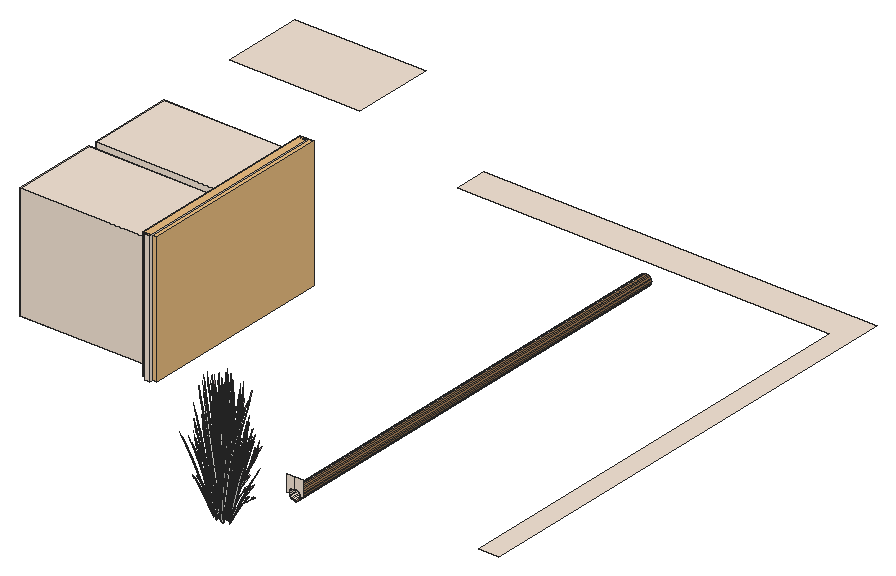
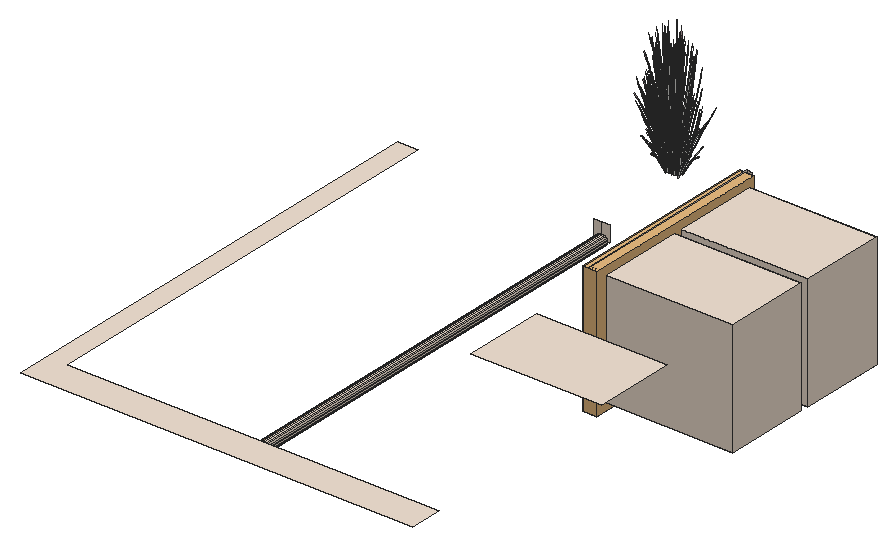
# SketchUp Ruby script. Lengths in inches.
U = 1.inch
M = Sketchup.active_model
def pt(a) = Geom::Point3d.new(a.map { |v| v * U })
def face(e, loops, mat)
  f = e.add_face(loops[0].map { |a| pt(a) })
  loops[1..].each { |l| e.add_face(l.map { |a| pt(a) }).erase! }
  f.material = f.back_material = mat if mat
  f
end
# faces: each face lists its corners as indices into pts; further lists are holes
def faces(e, pts, list, mat = nil) = list.each { |f| face(e, (f[0].is_a?(Array) ? f : [f]).map { |l| l.map { |i| pts[i] } }, mat) }
# xy, xz, yz: faces in a plane at the given z, y or x. An outline is a flat list of corners, or four numbers for a rectangle; further outlines are holes
def ring(l) = l.size == 4 ? [[l[0], l[1]], [l[2], l[1]], [l[2], l[3]], [l[0], l[3]]] : l.each_slice(2).to_a
def flat(e, list, mat, &to3) = list.each { |f| face(e, (f[0].is_a?(Array) ? f : [f]).map { |l| ring(l).map { |u, v| to3.(u, v) } }, mat) }
def xy(e, z, list, mat = nil) = flat(e, list, mat) { |x, y| [x, y, z] }
def xz(e, y, list, mat = nil) = flat(e, list, mat) { |x, z| [x, y, z] }
def yz(e, x, list, mat = nil) = flat(e, list, mat) { |y, z| [x, y, z] }
def lines(e, pts, list) = list.each { |a, b| e.add_line(pt(pts[a]), pt(pts[b])) }
# prism: a flat outline (further loops are holes) pulled along v
def prism(e, loops, v, mat = nil)
  f = face(e, loops, mat); d = Geom::Vector3d.new(v.map { |x| x * U })
  f.pushpull(f.normal.samedirection?(d) ? d.length : -d.length)
end
def box(e, o, s, mat = nil) = prism(e, [[o, [o[0] + s[0], o[1], o[2]], [o[0] + s[0], o[1] + s[1], o[2]], [o[0], o[1] + s[1], o[2]]]], [0, 0, s[2]], mat)
def at(x, y, z, deg = 0) = Geom::Transformation.translation(pt([x, y, z])) * Geom::Transformation.rotation(ORIGIN, Z_AXIS, deg.degrees)
def axes(o, x, y, z) = Geom::Transformation.new([*x, 0, *y, 0, *z, 0, *pt(o).to_a, 1])
def part(name) = M.definitions.add(name)
# library, detail: a bought-in or finely detailed component or shape, given as its bounding box
def library(name, o, s) = part(name).tap { |d| box(d.entities, o, s) }
def detail(e, o, s) = box(e.add_group.entities, o, s)
def put(e, d, t, mat = nil) = e.add_instance(d, t).tap { |i| i.material = mat if mat }
def group(e, t, mat = nil) = e.add_group.tap { |g| g.transformation = t; g.material = mat if mat }.entities
root = M.entities
M.materials.add("C01_Vanilla_Cream").color = [244, 228, 212]
M.materials.add("LightPink_Translucent").color = [144, 107, 117]
M.materials["LightPink_Translucent"].alpha = 0.75
M.materials.add("Wood_Floor_01_1K").color = [146, 111, 76]
c1 = part("blade")
p = [[2.15,0.21,22],[0,0.17,0],[0.09,0.45,0],[2.18,0.31,22],[2.29,0.31,22],[0.38,0.45,0],
  [2.48,0.24,33],[2.49,0.24,33],[2.48,0.22,33]]
faces(c1.entities,p,[[0,1,2,3],[4,5,2,3],[6,3,4,7],[8,0,3,6]])
c2 = part("seeds")
p = [[0.3,-0.1,1.38],[-0.01,-0.03,1.59],[-0.01,-0.03,0.03],[0.14,-0.07,-0.07],[0.29,-0.03,3],[0.15,0.01,3.11]]
faces(c2.entities,p,[[0,1,2,3],[1,0,4,5]],"LightPink_Translucent")
c3 = part("blade with seeds")
put(c3.entities,c1,at(0,0,0))
put(c3.entities,c2,axes([2.4,0.25,30.99],[1.5799,-0.05474,1.17369],[-0.12525,1.92788,0.29478],[-0.07173,-0.02425,1.56792]))
c4 = library("Double casement window",[0,0,0],[5.02,56.42,60])
xy(root,48,[[424.7,306.76,432,306.76,432,480,288,480,288,468,424.7,468],[288,324,290,396]],"C01_Vanilla_Cream")
xy(root,51,[[240,327,290,358.5],[240,361.5,290,393]],"C01_Vanilla_Cream")
xy(root,93,[[240,327,290,358.5],[240,361.5,290,393],[240,423,288,453]],"C01_Vanilla_Cream")
xz(root,306.76,[[354,42,354,48,357,48,357,44,356.48,43.93,356,43.73,355.59,43.41,355.27,43,355.07,42.52,355,42],[359,42,358.93,42.52,358.73,43,358.41,43.41,358,43.73,357.52,43.93,357,44,357,48,360,48,360,42]],"C01_Vanilla_Cream")
xz(root,324,[[288,48,290,96]],"C01_Vanilla_Cream")
xz(root,327,[[240,51,290,93]],"C01_Vanilla_Cream")
xz(root,358.5,[[240,51,290,93]],"C01_Vanilla_Cream")
xz(root,361.5,[[240,51,290,93]],"C01_Vanilla_Cream")
xz(root,393,[[240,51,290,93]],"C01_Vanilla_Cream")
xz(root,396,[[288,48,290,96]],"C01_Vanilla_Cream")
yz(root,240,[[327,51,358.5,93],[361.5,51,393,93]],"C01_Vanilla_Cream")
yz(root,290,[[[324,48,396,96],[327,51,358.5,93],[361.5,51,393,93]]],"C01_Vanilla_Cream")
p = [[357,306.76,40],[356.48,306.76,40.07],[356.48,468,40.07],[357,468,40],[357.52,306.76,40.07],[357.52,468,40.07],
  [356,306.76,40.27],[356,468,40.27],[358,306.76,40.27],[358,468,40.27],[355.59,306.76,40.59],[355.59,468,40.59],
  [358.41,306.76,40.59],[358.41,468,40.59],[355.27,306.76,41],[355.27,468,41],[358.73,306.76,41],[358.73,468,41],
  [355.07,306.76,41.48],[355.07,468,41.48],[358.93,306.76,41.48],[358.93,468,41.48],[355,306.76,42],[355,468,42],
  [359,306.76,42],[359,468,42],[355.07,306.76,42.52],[355.07,468,42.52],[358.93,306.76,42.52],[358.93,468,42.52],
  [355.27,306.76,43],[355.27,468,43],[358.73,306.76,43],[358.73,468,43],[355.59,306.76,43.41],[355.59,468,43.41],
  [358.41,306.76,43.41],[358.41,468,43.41],[356,306.76,43.73],[356,468,43.73],[358,306.76,43.73],[358,468,43.73],
  [356.48,306.76,43.93],[356.48,468,43.93],[357.52,306.76,43.93],[357.52,468,43.93],[357,306.76,44],[357,468,44]]
faces(root,p,[[0,1,2,3],[1,6,7,2],[6,10,11,7],[10,14,15,11],[14,18,19,15],[18,22,23,19],[22,26,27,23],[26,30,31,27],
  [30,34,35,31],[34,38,39,35],[38,42,43,39],[42,46,47,43]],"C01_Vanilla_Cream")
faces(root,p,[[4,0,3,5],[8,4,5,9],[12,8,9,13],[16,12,13,17],[20,16,17,21],[24,20,21,25],[28,24,25,29],[32,28,29,33],
  [36,32,33,37],[40,36,37,41],[44,40,41,45],[46,44,45,47]],"Wood_Floor_01_1K")
put(root,c3,axes([359.9,272.88,51.78],[-0.28012,-0.44611,-0.0912],[0.49717,-0.21923,-0.50621],[0.20951,-0.05886,0.76918]))
put(root,c3,axes([359.88,272.5,51.51],[0.15083,-0.44814,-0.38324],[0.51712,0.15361,-0.29685],[0.2082,-0.04109,0.7333]))
put(root,c3,axes([359.0625,270.67,49.78],[0.34808,-0.49367,0],[0.58235,0.27531,-0.38706],[0.13264,0.0627,1.22783]))
put(root,c3,axes([354.96,271.65,50.91],[0.23093,-0.01116,1.28532],[-0.15319,0.4836,0.10393],[-0.32909,-0.02991,0.54946]))
put(root,c3,axes([356.98,272.78,49.66],[-0.33445,-0.41351,-0.33554],[0.50659,-0.29119,0.16149],[-0.10823,-0.05117,1.07733]))
put(root,c3,axes([357.05,272.2,49.77],[0.24206,0.5509,0.34316],[-0.69162,0.19157,0.13466],[0.00845,-0.10123,1.19142]))
put(root,c3,axes([360.43,272.625,49.49],[-0.35858,0.05912,1.06187],[-0.05708,-0.47061,0.06078],[0.25115,-0.07123,0.60425]))
put(root,c3,axes([361.08,272.21,49.7],[-0.34516,-0.31503,-0.04866],[0.37803,-0.28865,-0.22062],[0.10711,-0.02032,0.72768]))
put(root,c3,axes([356.92,272.63,50.04],[-0.27012,0.44393,0.33554],[-0.56127,-0.21365,-0.16149],[0,-0.10233,1.07733]))
put(root,c3,axes([357.92,272.25,49.65],[0,-0.57005,0],[0.69617,0,0],[0,0,1.34592]))
put(root,c3,axes([358.76,270.93,49.86],[-0.52105,-0.24633,0.37238],[0.31144,-0.44171,0],[0.11867,0.0561,1.18128]))
put(root,c3,axes([359.78,272.66,51.74],[0.48922,-0.21758,-0.53284],[0.27264,0.44789,0.0643],[0.23638,-0.05088,0.75375]))
put(root,c3,axes([356.68,272.94,49.54],[-0.57914,-0.08077,-0.46765],[0.12221,-0.49823,-0.12274],[-0.17283,-0.06037,1.03225]))
put(root,c3,axes([357.59,271.89,49.77],[-0.46162,0.4471,0.34316],[-0.54842,-0.39467,0.13466],[0.11129,-0.04462,1.19142]))
put(root,c3,axes([358.09,272.6875,49.72],[-0.51786,-0.42404,-0.04598],[0.51817,-0.4243,0],[-0.01808,-0.01481,1.31678]))
put(root,c3,axes([356.79,271.15,49.86],[-0.16083,0.48962,0.13232],[-0.58854,-0.13856,0.26315],[0.10167,-0.00238,1.20305]))
put(root,c3,axes([359.71,272.75,51.79],[-0.46269,-0.13744,0.2656],[0.13495,-0.40096,-0.3429],[0.18628,-0.03677,0.65611]))
put(root,c3,axes([354.86,272.01,51.55],[0.15729,-0.44921,0.36002],[0.51712,0.15361,0.29685],[-0.20336,0.027,0.74497]))
put(root,c3,axes([356.54,271.55,49.2],[-0.548,0.19724,0.96696],[-0.17442,-0.56594,0.37572],[0.3365,0.00941,1.09981]))
put(root,c3,axes([358.01,271.7,49.96],[0.1074,-0.43968,0.1086],[0.52474,0.07632,-0.3101],[0.0955,0.04515,0.95058]))
put(root,c3,axes([354.83,271.89,51.55],[-0.20448,-0.33592,0.04823],[0.37288,-0.16442,0.37966],[-0.16437,0.03244,0.57892]))
put(root,c3,axes([357.11,272.74,49.77],[0.70367,0.1038,0.34316],[-0.1432,0.58624,0.13466],[-0.10283,-0.05661,1.19142]))
put(root,c3,axes([360.82,272.32,49.12],[-0.0291,-0.0748,1.32257],[0.20181,-0.43752,-0.20205],[0.20357,-0.00629,0.22528]))
put(root,c3,axes([354.81,272.24,49.12],[0.01412,0.07764,1.32257],[-0.28464,0.40547,-0.20205],[-0.20218,-0.02044,0.22528]))
put(root,c3,axes([357.79,271.8125,50.04],[-0.33445,-0.41351,0.33554],[0.50659,-0.29119,-0.16149],[0.10823,0.05117,1.07733]))
put(root,c3,axes([356.0625,273.7,49.52],[-0.13078,-0.42928,-0.23233],[0.51941,-0.1219,0.23233],[-0.10471,-0.0495,1.0423]))
put(root,c3,axes([356.73,273.68,49.86],[0.59825,-0.13076,0.13232],[0.14773,0.48663,0.26315],[-0.05336,-0.0709,1.20305]))
put(root,c3,axes([357.96,271.84,50],[0.56211,-0.32708,-0.21822],[0.3738,0.46216,-0.37502],[0.13869,0.04694,1.19781]))
put(root,c3,axes([360.2,272.7,51.39],[0.46269,0.13744,-0.2656],[-0.13495,0.40096,0.3429],[0.18628,-0.03677,0.65611]))
put(root,c3,axes([355.92,273.89,49.51],[-0.52105,-0.24633,-0.37238],[0.31144,-0.44171,0],[-0.11867,-0.0561,1.18128]))
put(root,c3,axes([359.38,270.97,49.51],[0.52105,0.24633,-0.37238],[-0.31144,0.44171,0],[0.11867,0.0561,1.18128]))
put(root,c3,axes([354.76,272.0625,51.39],[-0.46269,-0.13744,-0.2656],[0.13495,-0.40096,0.3429],[-0.18628,0.03677,0.65611]))
put(root,c3,axes([358.39,272.375,49.65],[0.62289,0,0],[0,0.51004,0],[0,0,1.33805]))
put(root,c3,axes([357.33,273.02,50],[-0.56211,0.32708,-0.21822],[-0.3738,-0.46216,-0.37502],[-0.13869,-0.04694,1.19781]))
put(root,c3,axes([358.57,271.18,49.86],[-0.59825,0.13076,0.13232],[-0.14773,-0.48663,0.26315],[0.05336,0.0709,1.20305]))
put(root,c3,axes([358.93,272.21,50.91],[-0.23093,0.01116,1.28532],[0.15319,-0.4836,0.10393],[0.32909,0.02991,0.54946]))
put(root,c3,axes([359.23,271.15,49.52],[0.13078,0.42928,-0.23233],[-0.51941,0.1219,0.23233],[0.10471,0.0495,1.0423]))
put(root,c3,axes([360.13,272.87,51.55],[0.20448,0.33592,0.04823],[-0.37288,0.16442,0.37966],[0.16437,-0.03244,0.57892]))
put(root,c3,axes([358.1875,272.12,49.79],[-0.70367,-0.1038,0.36899],[0.1432,-0.58624,0.1448],[0.10283,0.05661,1.2811]))
put(root,c3,axes([360.09,272.75,51.55],[-0.15729,0.44921,0.36002],[-0.51712,-0.15361,0.29685],[0.20336,-0.027,0.74497]))
put(root,c3,axes([357.625,273.5625,49.65],[-0.18165,-0.42474,0],[0.51872,-0.14874,0],[0,0,1.15778]))
put(root,c3,axes([357.28,273.16,49.96],[-0.1074,0.43968,0.1086],[-0.52474,-0.07632,-0.3101],[-0.0955,-0.04515,0.95058]))
put(root,c3,axes([355.24,272.02,51.79],[0.46269,0.13744,0.2656],[-0.13495,0.40096,-0.3429],[-0.18628,0.03677,0.65611]))
put(root,c3,axes([358.31,273.5,49.64],[0.5845,-0.16716,-0.14398],[0.20539,0.48152,0.00006],[0.06452,-0.01848,1.30423]))
put(root,c3,axes([358.51,273.7,49.86],[0.16083,-0.48962,0.13232],[0.58854,0.13856,0.26315],[-0.10167,0.00238,1.20305]))
put(root,c3,axes([358.375,272.59,49.66],[0.38863,0.31822,0],[-0.38863,0.31822,0],[0,0,1.2695]))
put(root,c3,axes([356.17,272,50.51],[0.15825,-0.07127,1.32798],[0.05457,0.4976,0.10393],[-0.34278,0.06603,0.47463]))
put(root,c3,axes([359.43,272.45,49.86],[-0.43742,-0.35886,0.13232],[0.44081,-0.34807,0.26315],[-0.04831,0.07329,1.20305]))
put(root,c3,axes([358.62,271.91,49.54],[0.57914,0.08077,-0.46765],[-0.12221,0.49823,-0.12274],[0.17283,0.06037,1.03225]))
put(root,c3,axes([361.18,272.78,50.07],[-0.34399,0.08133,0.86145],[0.16192,-0.33614,0.63294],[0.18249,0.023,0.18974]))
put(root,c3,axes([357.5,273.75,49.65],[-0.56127,-0.22118,0],[0.27012,-0.45959,0],[0,0,1.2203]))
put(root,c3,axes([357.96,273.17,49.85],[-0.54364,-0.39653,-0.18894],[0.45745,-0.44527,0.41347],[-0.14639,0.04639,1.26162]))
put(root,c3,axes([356.53,273.93,49.86],[0.52105,0.24633,0.37238],[-0.31144,0.44171,0],[-0.11867,-0.0561,1.18128]))
put(root,c3,axes([358.37,272.22,50.04],[0.27012,-0.44393,0.33554],[0.56127,0.21365,-0.16149],[0,0.10233,1.07733]))
put(root,c3,axes([361.02,274.21,51.53],[-0.05034,-0.04313,1.33037],[0.11012,-0.46232,-0.12571],[0.1983,-0.02954,0.23543]))
put(root,c3,axes([354.47,272.33,51.54],[-0.09091,0.06396,1.31208],[0.00773,0.46734,-0.2075],[-0.20839,0.06078,0.10523]))
put(root,c3,axes([358.27,272.48,49.72],[0,0.56976,-0.04228],[-0.69617,0,0],[0,0.01791,1.34526]))
put(root,c3,axes([355.07,272.27,51.51],[-0.15083,0.44814,-0.38324],[-0.51712,-0.15361,-0.29685],[-0.2082,0.04109,0.7333]))
put(root,c3,axes([355.05,271.88,51.78],[0.28012,0.44611,-0.0912],[-0.49717,0.21923,-0.50621],[-0.20951,0.05886,0.76918]))
put(root,c3,axes([358.32,272.07,49.66],[0.33445,0.41351,-0.33554],[-0.50659,0.29119,0.16149],[0.10823,0.05117,1.07733]))
put(root,c3,axes([360.58,273.82,50.95],[-0.10656,-0.41414,-0.02619],[0.50364,-0.09521,-0.11874],[0.10517,0.02626,0.39164]))
put(root,c3,axes([356.23,274.18,49.78],[-0.34808,0.49367,0],[-0.58235,-0.27531,-0.38706],[-0.13264,-0.0627,1.22783]))
put(root,c3,axes([359.27,273.81,51.78],[0.02981,-0.50103,-0.0912],[0.56442,0.01369,-0.50621],[0.21738,0.0348,0.76918]))
put(root,c3,axes([359.79,272.47,49.86],[0,-0.49266,0.37238],[0.62289,0,0],[0,0.11221,1.18128]))
put(root,c3,axes([358.23,272.84,50.04],[0.60457,-0.03041,0.33554],[0.05467,0.50484,-0.16149],[-0.10823,0.05117,1.07733]))
put(root,c3,axes([358.6,272.32,49.96],[0.51872,-0.14368,0.1086],[0.18165,0.41027,-0.3101],[0,0.09029,0.95058]))
put(root,c3,axes([359.1875,273.61,51.79],[-0.31678,-0.30846,0.2656],[0.36171,-0.29199,-0.3429],[0.18378,0.04443,0.65611]))
put(root,c3,axes([357.6875,273.08,49.66],[-0.60457,0.03041,-0.33554],[-0.05467,-0.50484,0.16149],[-0.10823,0.05117,1.07733]))
put(root,c3,axes([360.53,273.32,49.94],[-0.13408,-0.12117,1.07251],[0.17446,-0.40083,-0.23066],[0.27128,0.0543,0.45856]))
put(root,c3,axes([358.14,273.76,49.65],[0.56127,0.22118,0],[-0.27012,0.45959,0],[0,0,1.31215]))
put(root,c3,axes([359.76,273.51,51.54],[0.11943,-0.00833,1.31208],[0.32759,-0.38275,-0.2075],[0.21244,0.05052,0.10523]))
put(root,c3,axes([358.36,274.25,49.64],[-0.34375,-0.4954,-0.03857],[0.58235,-0.27531,0.38706],[-0.1435,0.04717,1.22723]))
put(root,c3,axes([358.24,273.05,49.96],[0.41131,0.296,0.1086],[-0.34309,0.33395,-0.3101],[-0.0955,0.04515,0.95058]))
put(root,c3,axes([354.99,273.13,51.55],[-0.13808,-0.45342,0.36002],[0.54163,-0.07869,0.29685],[-0.15963,0.10664,0.74497]))
put(root,c3,axes([354.88,273.04,51.55],[-0.3822,-0.20719,0.04823],[0.22252,-0.29505,0.37966],[-0.12254,0.09539,0.57892]))
put(root,c3,axes([355.06,272.5,50.91],[0.19317,-0.10421,1.28532],[0.16263,0.48153,0.10393],[-0.30326,0.10883,0.54946]))
put(root,c3,axes([359.3,273.57,51.74],[0.55654,0.01186,-0.53284],[-0.03738,0.49951,0.0643],[0.23578,0.05271,0.75375]))
put(root,c3,axes([358.67,273.97,49.86],[0.52105,-0.24633,0.37238],[0.31144,0.44171,0],[-0.11867,0.0561,1.18128]))
put(root,c3,axes([357.93,273.58,49.72],[0.24206,0.56598,-0.04509],[-0.69162,0.19832,0],[0.00845,0.01976,1.2913]))
put(root,c3,axes([358.2,274.19,49.52],[-0.51941,-0.1219,-0.23233],[0.13078,-0.42928,0.23233],[-0.10471,0.0495,1.0423]))
put(root,c3,axes([354.45,273.32,49.94],[0.19348,0.04044,1.07251],[0.1247,0.41309,-0.23066],[-0.26282,0.07733,0.45856]))
put(root,c3,axes([355.32,272.98,51.79],[0.48462,-0.07041,0.2656],[0.12797,0.4025,-0.3429],[-0.13888,0.10811,0.65611]))
put(root,c3,axes([360.21,272.55,49.78],[0.69617,0,0],[0,0.55062,-0.38706],[0,0.12541,1.22783]))
put(root,c3,axes([353.46,272.8,51.53],[0.07105,0.01321,1.33037],[0.2198,0.43529,-0.12571],[-0.14545,0.11425,0.23543]))
put(root,c3,axes([359.93,272.84,49.65],[-0.69582,-0.00394,-0.03732],[0,-0.55062,0.37457],[-0.02187,0.12535,1.18764]))
put(root,c3,axes([358.43,272.36,50],[0.62699,0.23507,-0.21822],[-0.3019,0.49615,-0.37502],[0.0197,0.12182,1.19781]))
put(root,c3,axes([354.05,274.18,50.07],[0.23202,-0.22328,0.86145],[0.09155,0.35348,0.63294],[-0.16768,0.06329,0.18974]))
put(root,c3,axes([359.64,273.77,51.39],[0.31678,0.30846,-0.2656],[-0.36171,0.29199,0.3429],[0.18378,0.04443,0.65611]))
put(root,c3,axes([359.79,272.92,49.52],[-0.38863,0.30738,-0.23233],[-0.38863,-0.30738,0.23233],[0,0.09901,1.0423]))
put(root,c3,axes([358.11,272.95,50],[0.06488,0.56215,-0.21822],[-0.6757,0.03399,-0.37502],[-0.11898,0.07488,1.19781]))
put(root,c3,axes([359.47,273.89,51.55],[-0.02803,0.37463,0.04823],[-0.42332,-0.01027,0.37966],[0.16216,0.0392,0.57892]))
put(root,c3,axes([358.36,272.73,49.66],[-0.27012,0.44393,-0.33554],[-0.56127,-0.21365,0.16149],[0,0.10233,1.07733]))
put(root,c3,axes([354.93,273.22,51.39],[-0.48462,0.07041,-0.2656],[-0.12797,-0.4025,0.3429],[-0.13888,0.10811,0.65611]))
put(root,c3,axes([359.51,273.77,51.55],[-0.41051,0.32462,0.36002],[-0.35404,-0.34474,0.29685],[0.1926,0.05988,0.74497]))
put(root,c3,axes([354.22,274.125,52.23],[0.49129,0.13151,-0.04866],[-0.15113,0.40475,-0.22062],[-0.08035,0.06145,0.72768]))
put(root,c3,axes([357.71,273.375,49.54],[-0.375,0.3703,-0.46765],[-0.46584,-0.33578,-0.12274],[-0.15027,0.09237,1.03225]))
put(root,c3,axes([358.21,274.15,51.79],[-0.08599,-0.39682,0.2656],[0.49155,-0.10478,-0.3429],[0.13203,0.11372,0.65611]))
put(root,c3,axes([358.375,274,49.75],[0.697,0.16013,0.23067],[-0.17437,0.57237,-0.27369],[-0.11536,0.07164,1.23664]))
put(root,c3,axes([358.32,274.38,49.51],[-0.52105,0.24633,-0.37238],[-0.31144,-0.44171,0],[-0.11867,0.0561,1.18128]))
put(root,c3,axes([360.06,272.93,49.51],[0,0.49266,-0.37238],[-0.62289,0,0],[0,0.11221,1.18128]))
put(root,c3,axes([358.5,272.98,50.91],[-0.2068,-0.08488,1.28532],[0.42797,-0.35609,0.10393],[0.26673,0.16064,0.54946]))
put(root,c3,axes([358.54,271.86,51.36],[-0.48108,-0.25598,1.03712],[0.50798,-0.39855,0.44749],[0.15521,0.24018,1.00248]))
put(root,c3,axes([355.07,272.94,51.78],[0.515,0.27165,-0.0912],[-0.2967,0.3934,-0.50621],[-0.1455,0.13675,0.76918]))
put(root,c3,axes([359.26,273.95,50.07],[-0.31347,-0.14166,0.86145],[0.40476,-0.14393,0.63294],[0.10917,0.12192,0.18974]))
put(root,c3,axes([358.16,274.35,51.78],[0.33176,-0.4217,-0.0912],[0.48044,0.24295,-0.50621],[0.16701,0.11914,0.76918]))
put(root,c3,axes([355.76,272.82,50.91],[0.13906,-0.15138,1.28532],[0.35111,0.40859,0.10393],[-0.24082,0.18608,0.54946]))
put(root,c3,axes([355.33,273.27,51.51],[0.14302,0.44985,-0.38324],[-0.54163,0.07869,-0.29685],[-0.15522,0.12083,0.7333]))
put(root,c3,axes([355.98,273.78,51.79],[0.3767,-0.25939,0.2656],[0.3566,0.29618,-0.3429],[-0.05426,0.15048,0.65611]))
put(root,c3,axes([358.8,274.31,49.78],[0.34808,0.49367,0],[-0.58235,0.27531,-0.38706],[-0.13264,0.0627,1.22783]))
put(root,c3,axes([357.73,274.7,51.53],[0.00165,-0.05965,1.33037],[0.47711,-0.26315,-0.12571],[0.16572,0.09393,0.23543]))
put(root,c3,axes([359.35,274.47,49.12],[0.04056,-0.07113,1.32257],[0.51066,-0.20948,-0.20205],[0.15482,0.10842,0.22528]))
put(root,c3,axes([358.5,272.35,50.13],[-0.01521,-0.46386,1.05954],[0.68831,0.12024,0.44862],[-0.1628,0.25382,1.00012]))
put(root,c3,axes([358.68,272.86,49.57],[0.20414,0.45107,-0.51909],[-0.58805,0.16245,-0.13624],[0.02256,0.15274,1.1458]))
put(root,c3,axes([355.63,274.02,51.55],[-0.45752,-0.02296,0.04823],[0.01254,-0.34663,0.37966],[-0.04787,0.13278,0.57892]))
put(root,c3,axes([354.66,274.41,49.12],[0.07468,0.04922,1.32257],[0.12663,0.45605,-0.20205],[-0.16551,0.09725,0.22528]))
put(root,c3,axes([355.78,274.05,51.55],[-0.39645,-0.33614,0.36002],[0.42102,-0.2899,0.29685],[-0.07313,0.15771,0.74497]))
put(root,c3,axes([358.56,274.14,51.51],[0.54938,-0.11711,-0.38324],[0.0961,0.44351,-0.29685],[0.14756,0.1271,0.7333]))
put(root,c3,axes([357.03,274.21,51.79],[0.16784,-0.37886,0.2656],[0.48968,0.1105,-0.3429],[0.0449,0.15254,0.65611]))
put(root,c3,axes([359.3125,274.59,50],[-0.35702,-0.01545,0.78795],[0.23577,-0.32816,0.43504],[0.14104,0.11659,0.61808]))
put(root,c3,axes([358.29,274.51,51.55],[-0.25304,0.31296,0.04823],[-0.36033,-0.18221,0.37966],[0.11649,0.10034,0.57892]))
put(root,c3,axes([357.69,275.5625,52.23],[0.38473,-0.28263,-0.04866],[0.35252,0.30954,-0.22062],[0.02482,0.08771,0.72768]))
put(root,c3,axes([358.39,274.42,51.55],[-0.55374,0.11306,0.36002],[-0.0961,-0.44351,0.29685],[0.13023,0.13071,0.74497]))
put(root,c3,axes([355.66,273.2,50.91],[0.10366,-0.16934,1.28532],[0.43488,0.35044,0.10393],[-0.19618,0.21841,0.54946]))
put(root,c3,axes([358.15,273.8,49.94],[0.00982,-0.16331,1.07251],[0.4695,-0.18242,-0.23066],[0.14493,0.19547,0.45856]))
put(root,c3,axes([356.88,274.55,51.55],[-0.41024,0.16744,0.04823],[-0.2008,-0.30532,0.37966],[0.03962,0.13459,0.57892]))
put(root,c3,axes([355.78,274.15,51.39],[-0.3767,0.25939,-0.2656],[-0.3566,-0.29618,0.3429],[-0.05426,0.15048,0.65611]))
put(root,c3,axes([354.48,274.07,51.54],[-0.01384,0.09749,1.31208],[0.39274,0.33916,-0.2075],[-0.10282,0.16039,0.10523]))
put(root,c3,axes([355.74,273.85,52.05],[0.61188,0.02441,-0.10123],[-0.01672,0.46217,-0.56189],[-0.0425,0.178,0.85379]))
put(root,c3,axes([356.87,274.37,51.78],[0.54481,-0.22937,-0.0912],[0.26773,0.4071,-0.50621],[0.07188,0.17155,0.76918]))
put(root,c3,axes([357.03,274.52,51.8],[-0.54859,-0.1288,0.39962],[0.18759,-0.42344,0.32951],[0.03297,0.16652,0.82692]))
put(root,c3,axes([356.02,275.16,50.07],[-0.01441,-0.29294,0.86145],[0.36003,0.20894,0.63294],[-0.07081,0.13963,0.18974]))
put(root,c3,axes([356.97,274.46,49.12],[0.0901,-0.02681,1.32257],[0.54199,0.14755,-0.20205],[0.01585,0.1663,0.22528]))
put(root,c3,axes([356.15,274.03,51.75],[0.39855,0.33102,-0.4254],[-0.42102,0.2899,-0.32951],[-0.06064,0.16819,0.81396]))
put(root,c3,axes([355.72,274.53,50.12],[0.50577,-0.08724,0.04881],[0.11627,0.35148,-0.64728],[-0.03206,0.17792,0.5802]))
put(root,c3,axes([357.34,274.35,51.51],[0.54728,0.1235,-0.38324],[-0.18759,0.42344,-0.29685],[0.05018,0.17048,0.7333]))
put(root,c3,axes([357.65,273.48,50.91],[-0.12726,-0.15818,1.28532],[0.58807,-0.13317,0.10393],[0.13291,0.24832,0.54946]))
put(root,c3,axes([357.09,274.61,51.39],[-0.16784,0.37886,-0.2656],[-0.48968,-0.1105,0.3429],[0.0449,0.15254,0.65611]))
put(root,c3,axes([356.03,273.875,52],[-0.01449,0.45571,-0.59145],[-0.61002,-0.03061,0.07138],[-0.06438,0.19306,0.83667]))
put(root,c3,axes([354.4375,275.07,51.53],[0.06316,-0.02974,1.33037],[0.52204,0.19785,-0.12571],[-0.01227,0.16473,0.23543]))
put(root,c3,axes([356.61,273.55,50.91],[-0.01363,-0.18909,1.28532],[0.5906,0.12544,0.10393],[-0.03653,0.26947,0.54946]))
put(root,c3,axes([357.14,274.27,51.74],[0.26572,0.40059,-0.53284],[-0.54698,0.22325,0.0643],[0.06214,0.19355,0.75375]))
put(root,c3,axes([355.6,274.9,49.94],[0.17569,-0.07772,1.07251],[0.43377,0.23434,-0.23066],[-0.12911,0.20277,0.45856]))
put(root,c3,axes([356.74,275.28,51.54],[0.07057,0.07933,1.31208],[0.56952,0.03117,-0.2075],[0.05727,0.17496,0.10523]))
put(root,c3,axes([355.83,274.52,50.52],[0.01223,-0.25433,1.15759],[0.55017,0.13434,0.15997],[-0.04767,0.27105,0.54661]))
put(root,c4,axes([286.7,325.0625,48.3],[1,0,0],[0,1.27666,0],[0,0,0.79394]))
